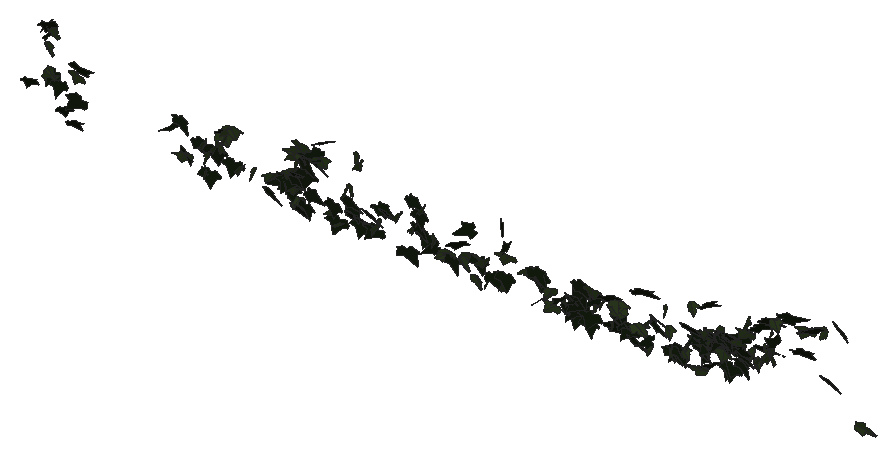
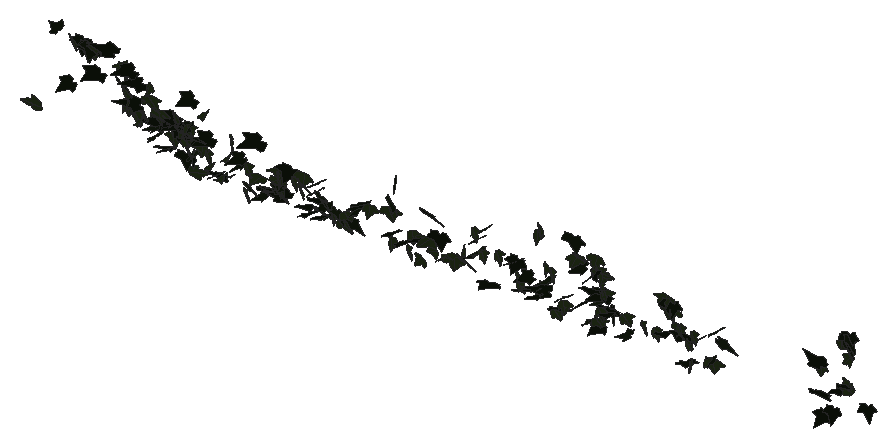
# SketchUp Ruby script. Lengths in millimetres.
U = 1.mm
M = Sketchup.active_model
def pt(a) = Geom::Point3d.new(a.map { |v| v * U })
def face(e, loops, mat)
  f = e.add_face(loops[0].map { |a| pt(a) })
  loops[1..].each { |l| e.add_face(l.map { |a| pt(a) }).erase! }
  f.material = f.back_material = mat if mat
  f
end
# faces: each face lists its corners as indices into pts; further lists are holes
def faces(e, pts, list, mat = nil) = list.each { |f| face(e, (f[0].is_a?(Array) ? f : [f]).map { |l| l.map { |i| pts[i] } }, mat) }
# xy, xz, yz: faces in a plane at the given z, y or x. An outline is a flat list of corners, or four numbers for a rectangle; further outlines are holes
def ring(l) = l.size == 4 ? [[l[0], l[1]], [l[2], l[1]], [l[2], l[3]], [l[0], l[3]]] : l.each_slice(2).to_a
def flat(e, list, mat, &to3) = list.each { |f| face(e, (f[0].is_a?(Array) ? f : [f]).map { |l| ring(l).map { |u, v| to3.(u, v) } }, mat) }
def xy(e, z, list, mat = nil) = flat(e, list, mat) { |x, y| [x, y, z] }
def xz(e, y, list, mat = nil) = flat(e, list, mat) { |x, z| [x, y, z] }
def yz(e, x, list, mat = nil) = flat(e, list, mat) { |y, z| [x, y, z] }
def lines(e, pts, list) = list.each { |a, b| e.add_line(pt(pts[a]), pt(pts[b])) }
# prism: a flat outline (further loops are holes) pulled along v
def prism(e, loops, v, mat = nil)
  f = face(e, loops, mat); d = Geom::Vector3d.new(v.map { |x| x * U })
  f.pushpull(f.normal.samedirection?(d) ? d.length : -d.length)
end
def box(e, o, s, mat = nil) = prism(e, [[o, [o[0] + s[0], o[1], o[2]], [o[0] + s[0], o[1] + s[1], o[2]], [o[0], o[1] + s[1], o[2]]]], [0, 0, s[2]], mat)
def at(x, y, z, deg = 0) = Geom::Transformation.translation(pt([x, y, z])) * Geom::Transformation.rotation(ORIGIN, Z_AXIS, deg.degrees)
def axes(o, x, y, z) = Geom::Transformation.new([*x, 0, *y, 0, *z, 0, *pt(o).to_a, 1])
def part(name) = M.definitions.add(name)
# library, detail: a bought-in or finely detailed component or shape, given as its bounding box
def library(name, o, s) = part(name).tap { |d| box(d.entities, o, s) }
def detail(e, o, s) = box(e.add_group.entities, o, s)
def put(e, d, t, mat = nil) = e.add_instance(d, t).tap { |i| i.material = mat if mat }
def group(e, t, mat = nil) = e.add_group.tap { |g| g.transformation = t; g.material = mat if mat }.entities
root = M.entities
M.materials.add("efeu1").color = [18, 25, 13]
M.materials.add("efeu2").color = [43, 57, 29]
c1 = part("ivyleaf_9")
p = [[39.1,54.8,31.7],[34.5,51.8,30.2],[-5.3,25.2,17.3],[-17.9,28.3,20.9],[-21.6,21.7,17],[-20.2,4.3,5.3],
  [-22.9,-0.3,2.5],[-17.1,-4,-0.6],[-2,-2.1,-1.2],[-0.7,-15.4,-10.1],[16.6,-22.3,-16.7],[21.1,-15.1,-12.5],
  [32.7,-10.7,-11],[46.1,-1.8,-6.6],[30.8,11.2,3.8]]
faces(c1.entities,p,[[0,1,2,3,4,5,6,7,8,9,10,11,12,13,14]],"efeu1")
c2 = part("ivyleaf_10")
p = [[0,12.8,-0.8],[-1.5,51.3,-10.9],[-4.9,51,-11.6],[-13.6,26.5,-7.3],[-13.2,15.9,-4.6],[-21.1,19.3,-7.2],
  [-29.5,16.3,-8.3],[-29.2,8.3,-6.2],[-19.7,-9.8,0.5],[-7.6,-13,4],[1,-12.2,5.8],[-0.4,51.1,-11.1],
  [-1.5,51.1,-10.9],[1,-12.4,5.9],[16.9,-12.4,3.5],[35.1,9.1,-5.1],[35,12.9,-6.1],[20.5,16.4,-4.9],
  [15.8,15,-3.8],[15.3,27.6,-7.1],[12.8,31.3,-7.8]]
faces(c2.entities,p,[[0,1,2,3,4,5,6,7,8,9,10],[11,12,0,13,14,15,16,17,18,19,20]],"efeu2")
put(root,c1,axes([3524.8,853.8,2688.6],[-0.38243,-1.02571,-0.0328],[-0.02604,0.0361,-1.04501],[1.95296,-0.20038,-0.02036]))
put(root,c2,axes([2249.2,836.8,2987.3],[-1.94583,0.29815,0.06081],[-0.10761,0.02331,-1.06497],[-0.56904,-1.02394,-0.00654]))
put(root,c2,axes([2960.6,842.6,2771.6],[-0.10375,-1.04241,-0.06639],[0.01698,0.06602,-1.04382],[1.98787,-0.05497,0.00545]))
put(root,c2,axes([5163.4,847,2805.5],[0.54884,-1.01393,0.11412],[0.04034,-0.11261,-1.05409],[1.94147,0.28897,-0.01036]))
put(root,c2,axes([3837.8,845,2630.1],[-1.522,0.00914,0.62017],[-1.11726,-0.33774,-0.75202],[0.38097,-0.95398,0.27218]))
put(root,c1,axes([3781,843.8,2662.2],[-0.77409,0.78081,-0.50896],[0.22007,-0.50875,-0.87289],[-1.76015,-0.40699,0.1147]))
put(root,c2,axes([2371.2,839.1,2946.3],[-1.56462,-0.61552,-0.30437],[0.59717,0.08559,-1.02058],[1.16244,-0.87245,0.11462]))
put(root,c1,axes([1819.8,855.8,2726.1],[-1.01559,-0.89248,-0.01376],[0.03018,0.00655,-1.03979],[1.69851,-0.53376,0.01024]))
put(root,c2,axes([5434.7,847.5,3054.3],[-1.65245,-0.47011,0.42813],[-0.52953,-0.37065,-0.97126],[1.08812,-0.8943,0.1775]))
put(root,c2,axes([2181.7,847.8,2815.4],[-0.62496,-0.9717,0.2211],[-0.05333,-0.22369,-1.02474],[1.89586,-0.32661,0.04406]))
put(root,c2,axes([840.3,839.1,2880.5],[-1.78166,0.36905,0.24353],[-0.53454,-0.05592,-0.99491],[-0.64994,-0.96568,0.15068]))
put(root,c2,axes([4806.6,848.5,2828],[-0.5462,-0.98923,0.23334],[-0.03803,-0.23693,-1.02901],[1.934,-0.28404,0.04567]))
put(root,c1,axes([5480,827.7,3079.3],[0.8704,0.9826,-0.02659],[-0.005,-0.02811,-1.08378],[-1.87077,0.45725,-0.00947]))
put(root,c2,axes([2720.9,851.5,2683.4],[0.06731,-0.98215,0.34089],[-0.00137,-0.34111,-0.98271],[1.97861,0.03318,-0.01228]))
put(root,c1,axes([4776.2,863.7,2677.8],[-0.34733,-0.64065,0.78184],[-0.14186,-0.78379,-0.65964],[1.91851,-0.17394,0.09277]))
put(root,c1,axes([3188,853.2,2671.4],[0.18907,-1.04431,-0.03336],[-0.04427,0.03129,-1.04883],[1.98806,0.10002,-0.02018]))
put(root,c1,axes([3320.6,844.8,2878.5],[-1.86535,0.38799,0.10195],[-0.1859,0.03022,-1.05409],[-0.74052,-0.98494,0.00782]))
put(root,c2,axes([1658.5,854.2,2723.5],[0.29167,-0.92037,0.46601],[0.22757,-0.45211,-0.93222],[1.95015,0.19041,0.03908]))
put(root,c2,axes([2741.6,841.1,2718.1],[0.53876,-0.97275,-0.25324],[-0.0295,0.25883,-1.01157],[1.91281,0.27797,0.05573]))
put(root,c2,axes([4220.5,854.1,2678.7],[0.20291,-0.93081,0.4596],[0.20811,-0.44938,-0.93547],[1.96471,0.14373,0.05162]))
put(root,c2,axes([4092.2,838.4,2805.9],[-1.96075,0.12903,0.14532],[-0.26905,0.04033,-1.03805],[-0.25379,-1.03965,-0.02224]))
put(root,c2,axes([5231.5,838.5,3036.9],[0.50163,1.03539,0.09613],[0.01258,0.0975,-1.06827],[-1.97899,0.26307,0.01758]))
put(root,c2,axes([5130.2,848.4,2783.3],[0.12425,-1.04507,0.14266],[0.00203,-0.14286,-1.04708],[2.00742,0.06483,-0.00777]))
put(root,c1,axes([721.9,857.1,2788],[-0.70151,-0.91712,-0.02718],[0.01443,0.02467,-1.08247],[1.11929,-0.57512,-0.00308]))
put(root,c1,axes([4004.6,854,2708.3],[-1.90405,-0.31834,0.02077],[-0.03708,-0.00727,-1.04987],[0.60602,-1.00064,0.00102]))
put(root,c2,axes([2524.7,841.7,2817.8],[0.33537,-1.02725,-0.2257],[0.01394,0.23004,-1.04128],[2.00165,0.17051,0.04506]))
put(root,c1,axes([5297.4,834.8,3075.8],[0.5679,-0.01909,1.03753],[1.97495,0.00564,-0.29834],[-0.00027,1.07957,0.0199]))
put(root,c1,axes([3964,856.5,2655.2],[-1.79592,-0.22886,-0.35753],[0.77032,-0.22235,-0.92594],[0.24355,-0.98429,0.2923]))
put(root,c2,axes([1769.1,844.1,2856.5],[0.40161,-1.0348,-0.11686],[0.03197,0.12261,-1.05532],[1.9817,0.20773,0.04071]))
put(root,c1,axes([2359.5,840.3,2956],[-1.405,0.61644,0.46097],[-0.92564,0.12149,-0.94136],[-1.13547,-0.86181,0.19702]))
put(root,c2,axes([5084.8,850.5,2813.4],[1.0935,-0.85291,0.23371],[0.30636,-0.17319,-1.02776],[1.65499,0.59561,0.03583]))
put(root,c1,axes([4909,855.7,2835.7],[0.28184,-1.02702,0.11184],[0.02485,-0.11111,-1.03764],[1.96603,0.14864,-0.00292]))
put(root,c1,axes([4766.3,858.5,2671.6],[-0.31118,0.09515,-1.0236],[1.52436,-0.63795,-0.18724],[-1.2265,-0.81702,0.02699]))
put(root,c2,axes([4706.2,841.7,2943.8],[0.18012,1.06557,-0.0634],[-0.03404,-0.06206,-1.06969],[-2.03129,0.09553,0.0123]))
put(root,c2,axes([3546,844.5,2807.2],[-1.80956,-0.35541,0.30029],[-0.49786,-0.15666,-1.01368],[0.73233,-0.98471,0.05289]))
put(root,c2,axes([3423.7,846,2629.2],[0.49046,-1.02396,-0.05486],[-0.00527,0.05587,-1.05584],[1.95159,0.25749,0.01093]))
put(root,c2,axes([4147.6,844.8,2765.4],[0.29206,-1.03516,-0.1201],[-0.05918,0.11679,-1.04638],[1.98245,0.15599,-0.01354]))
put(root,c1,axes([4835.8,831.1,2659.2],[0.53256,0.98286,-0.06512],[-0.06187,-0.05844,-1.02181],[-1.87366,0.28129,0.01523]))
put(root,c1,axes([2742.9,834.6,2799.4],[1.77656,0.12528,-0.48402],[-0.92454,-0.01528,-0.9408],[-0.22513,1.05137,0.04401]))
put(root,c1,axes([4952.1,859.3,2674.2],[-1.41903,-0.72291,-0.02914],[0.26822,-0.10407,-1.02405],[1.35058,-0.73888,0.17275]))
put(root,c1,axes([2478,857,2633.5],[-1.34236,-0.72939,-0.04705],[0.06489,0.03248,-1.01463],[1.38954,-0.70614,0.00193]))
put(root,c2,axes([4772.1,849.8,2593],[-0.5713,0.16608,-0.97809],[-1.87241,-0.18152,0.27112],[-0.24333,1.00689,0.21021]))
put(root,c2,axes([649.1,847.9,2983.9],[-0.91633,0.44988,-0.67449],[0.65762,-0.40971,-0.87353],[-0.73885,-0.92261,0.05902]))
put(root,c1,axes([4826.2,858.9,2792.3],[-0.76048,0.05698,-0.9592],[1.5315,-0.54789,-0.36777],[-0.99945,-0.88292,0.16631]))
put(root,c2,axes([4900.9,844,2746.7],[1.93704,-0.15175,-0.03007],[-0.00635,0.17855,-1.01386],[0.29435,1.00245,0.17603]))
put(root,c1,axes([4827,856.9,2759.9],[-1.70999,-0.50276,0.04313],[-0.08161,-0.0117,-1.02953],[0.95689,-0.89944,-0.01072]))
put(root,c1,axes([4770.9,852.1,2779.7],[-1.97824,-0.02307,0.01489],[-0.02887,0.01257,-1.03961],[0.04356,-1.03946,-0.01291]))
put(root,c1,axes([5242.8,828.7,2918],[-0.55871,0.81079,0.61449],[-0.48403,0.56077,-0.86141],[-1.87473,-0.38642,0.03927]))
put(root,c1,axes([4938.1,860.7,2666.4],[-0.47857,-0.98898,0.18704],[-0.00593,-0.19202,-1.01951],[1.91558,-0.24767,0.04357]))
put(root,c1,axes([3713.3,848.5,2787.9],[0.13317,-0.99633,-0.43816],[0.23105,0.44347,-0.98902],[2.05856,0.01468,0.13935]))
put(root,c1,axes([3991.1,855.7,2759],[0.10791,-1.02927,-0.01108],[0.05026,0.01255,-1.03047],[1.95837,0.05639,0.02705]))
put(root,c1,axes([4107.5,850.2,2772.3],[-1.68755,0.40318,-0.38442],[0.62497,-0.20543,-0.97289],[-0.85644,-0.94435,0.04751]))
put(root,c2,axes([4101,847.7,2732.1],[0.95268,-0.93252,-0.02492],[0.06155,0.04561,-1.05719],[1.77434,0.49911,0.05005]))
put(root,c1,axes([2982.2,860,2843.2],[-0.18743,-1.02006,0.18085],[-0.04885,-0.17921,-1.02477],[1.97105,-0.10144,-0.0082]))
put(root,c2,axes([5195.3,843.9,2825.3],[-0.33655,-1.03716,-0.15633],[-0.0239,0.16062,-1.0514],[1.99607,-0.17295,-0.03895]))
put(root,c2,axes([2600.2,841.7,3040.9],[0.94944,-0.8955,-0.3093],[-0.00123,0.34923,-1.01217],[1.80311,0.47177,0.16217]))
put(root,c1,axes([4051.6,857.4,2615],[-0.36566,-1.02505,-0.02846],[-0.01091,0.03003,-1.04284],[1.9516,-0.19189,-0.01117]))
put(root,c1,axes([4801.8,823.6,2981.8],[1.0595,0.6289,0.69898],[0.9003,0.51468,-0.83983],[-1.54653,0.73046,-0.01005]))
put(root,c1,axes([652.9,837.1,3113],[0.67461,0.83088,-0.50179],[-0.36156,-0.4054,-0.99787],[-1.12764,0.62706,0.01976]))
put(root,c2,axes([1866.2,849,2717],[-0.03693,-1.03805,0.06821],[-0.02331,-0.06799,-1.03817],[1.97974,-0.02017,-0.01095]))
put(root,c2,axes([4892.9,847.5,2866],[1.19897,-0.85151,-0.01828],[0.14211,0.07787,-1.05387],[1.61473,0.62541,0.10632]))
put(root,c2,axes([1631.8,847.4,2777.5],[0.15517,-1.04614,-0.0366],[0.00203,0.0368,-1.0493],[1.99223,0.08144,0.00392]))
put(root,c2,axes([1756.2,841.6,2862.7],[1.74782,0.41459,0.34556],[0.49005,0.26283,-0.99965],[-0.90276,0.94536,0.12638]))
put(root,c1,axes([847.3,856.1,2736.8],[-1.85697,-0.29641,0.05056],[-0.09128,-0.01608,-1.01974],[0.56495,-0.97689,0.00144]))
put(root,c1,axes([3521.7,825,2971],[0.1987,0.34296,-1.03239],[-1.72012,0.60458,0.10944],[1.15234,0.84333,0.34139]))
put(root,c2,axes([1803.7,839.9,2920.1],[1.88423,0.20389,0.3712],[0.53319,0.3925,-0.9628],[-0.60447,0.98179,0.30782]))
put(root,c1,axes([4205.4,837.6,2644.7],[0.56789,-0.08644,1.07907],[2.06015,0.01167,-0.29839],[0.02237,1.11951,0.08643]))
put(root,c2,axes([4996.3,843.5,2842.1],[-1.85555,0.00075,0.3707],[-0.70424,-0.06486,-0.97306],[0.04254,-1.04104,0.0609]))
put(root,c1,axes([4804.2,848.2,2828.9],[1.39993,-0.75627,0.08125],[0.24801,0.01394,-1.04997],[1.42622,0.73991,0.10283]))
put(root,c1,axes([5385.1,832,2928.8],[1.87767,0.38759,0.22071],[0.39423,0.07633,-1.05998],[-0.75178,1.00809,-0.0046]))
put(root,c2,axes([4556.7,848.4,2753.1],[0.18081,1.01006,-0.29537],[0.01311,-0.29716,-1.01397],[-2.00281,0.08924,-0.0333]))
put(root,c1,axes([4173.6,832.4,2808.1],[1.51407,0.6998,-0.06753],[-0.0701,-0.06035,-1.05932],[-1.33621,0.79612,-0.02094]))
put(root,c1,axes([2551.6,844.9,2695.3],[1.4633,-0.37434,0.60056],[1.13248,-0.13804,-0.84783],[0.72903,0.9658,0.11159]))
put(root,c2,axes([4237.1,845.3,2787.7],[1.5894,0.66517,-0.01359],[-0.11775,0.05593,-1.06448],[-1.26073,0.83336,0.08228]))
put(root,c1,axes([1470.1,854.8,2854.2],[0.38581,-1.02413,-0.08631],[-0.00857,0.08709,-1.04393],[1.95602,0.20238,0.01245]))
put(root,c1,axes([2710.6,864.3,2657.9],[-1.4816,-0.58663,0.29971],[-0.15276,-0.37605,-0.94453],[1.24441,-0.74461,0.24089]))
put(root,c1,axes([2967.4,852.3,2779.4],[0.72248,-0.97219,-0.12719],[-0.05329,0.12558,-1.04349],[1.86527,0.38015,0.01945]))
put(root,c2,axes([3251.8,854.7,2685.9],[-1.07715,0.43778,-0.75759],[0.86821,-0.62229,-0.7004],[-1.42103,-0.71205,0.14633]))
put(root,c2,axes([1939.7,854.3,2723.3],[0.68737,-1.00756,0.23911],[0.16631,-0.22267,-1.07031],[1.96382,0.37152,0.00695]))
put(root,c2,axes([5757.7,846.8,2623.9],[0.2653,-0.05489,1.12507],[2.12837,0.14239,-0.13161],[-0.25651,1.12469,0.07157]))
put(root,c2,axes([2489.2,855.6,2610.1],[-0.46165,-0.89885,0.38975],[-0.08079,-0.3915,-0.9293],[1.86284,-0.23973,0.05628]))
put(root,c1,axes([5551,840,2820.8],[1.99954,-0.28673,-0.22437],[-0.38922,0.10217,-1.08816],[0.57328,1.06944,0.0438]))
put(root,c2,axes([5054.3,846.8,2903.5],[-1.65578,-0.20003,0.54473],[-1.00179,-0.14123,-0.89254],[0.46493,-1.0167,0.01681]))
put(root,c1,axes([4901.1,837.5,2851.5],[2.00867,0.1427,-0.16912],[-0.31404,-0.0416,-1.06485],[-0.28059,1.06807,-0.01888]))
put(root,c2,axes([2857.7,849.7,2801.7],[-0.09278,-1.04773,0.01676],[0.02837,-0.01747,-1.04875],[1.9941,-0.0485,0.0157]))
put(root,c2,axes([5208.8,846.6,2895.4],[1.27296,-0.79938,-0.1908],[-0.06895,0.21709,-1.03651],[1.56261,0.66079,0.1097]))
put(root,c1,axes([4065.8,862.1,2653.8],[-1.2522,-0.79879,0.01773],[0.12516,-0.07703,-1.03005],[1.51547,-0.65366,0.09972]))
put(root,c1,axes([3091.1,849.7,2701.1],[-1.7001,0.47822,-0.14667],[0.20459,-0.10964,-1.01222],[-0.92975,-0.89858,0.04545]))
put(root,c1,axes([3970.3,862.3,2625.4],[-0.7348,-0.95523,0.09098],[-0.00188,-0.09768,-1.02969],[1.82622,-0.38445,0.03555]))
put(root,c2,axes([2197.9,839.9,2912.1],[-0.67537,-0.86746,-0.47866],[0.40694,0.4294,-0.93671],[1.84118,-0.41311,0.03145]))
put(root,c1,axes([2312.5,848,2918.4],[1.51589,-0.69692,-0.08546],[-0.11258,0.06217,-1.05832],[1.33155,0.79865,0.00781]))
put(root,c1,axes([4977.3,841.4,2793.4],[0.43064,0.09525,-1.03432],[1.52589,0.65699,0.2359],[1.25681,-0.83029,0.068]))
put(root,c2,axes([2212.4,846.9,2856.8],[0.44043,-1.01871,-0.1879],[-0.04046,0.18782,-1.04446],[1.9711,0.23148,0.02055]))
put(root,c1,axes([4848.1,857.2,2798],[-1.67592,-0.12919,-0.52249],[1.01319,-0.0616,-0.88199],[0.15078,-1.02206,0.1192]))
put(root,c1,axes([2390.5,832.5,3050],[0.56887,1.03665,-0.02085],[-0.32189,0.02734,-1.0654],[-1.94692,0.29838,0.17005]))
put(root,c1,axes([5443.3,833.2,3063.6],[0.59201,1.0353,-0.02549],[-0.04944,-0.0188,-1.08084],[-1.97035,0.31154,0.01946]))
put(root,c1,axes([4883.3,851.7,2828.8],[0.66188,-0.96398,-0.24228],[-0.00401,0.25597,-1.02145],[1.89169,0.33783,0.08261]))
put(root,c2,axes([1709.6,850.8,2786.3],[0.07885,-1.05163,0.02218],[-0.06371,-0.0235,-1.05188],[2.00089,0.04069,-0.03437]))
put(root,c2,axes([4683.4,848.8,2723.5],[0.26435,-1.04108,-0.08736],[0.04998,0.09158,-1.04962],[1.98773,0.13615,0.03801]))
put(root,c1,axes([2144.5,835.2,2738.1],[0.62374,-0.16783,-0.99526],[-1.7124,0.42556,-0.36805],[0.87039,0.95752,-0.01087]))
put(root,c1,axes([3982,830.4,2719.8],[-0.28066,0.85178,0.56979],[-0.37015,0.54193,-0.86048],[-1.91493,-0.2296,0.08282]))
put(root,c2,axes([4542.2,843.7,2859.6],[0.70772,-0.92594,-0.35762],[-0.01438,0.37924,-0.98978],[1.88907,0.34978,0.12645]))
put(root,c1,axes([4673.7,841.3,2812.7],[2.10002,-0.18849,-0.00836],[-0.01636,-0.00064,-1.1194],[0.35872,1.10345,-0.00208]))
put(root,c1,axes([2256.4,848.3,2894.6],[0.78631,-0.87903,-0.41991],[-0.39191,0.367,-0.97089],[1.81216,0.46079,-0.02777]))
put(root,c1,axes([671.4,841.4,3062],[-0.7447,0.92163,0.02249],[-0.01308,0.01987,-1.10544],[-1.12465,-0.6105,-0.00204]))
put(root,c1,axes([2652.5,846,2745.4],[1.80729,-0.4543,0.00246],[0.00416,-0.00113,-1.05268],[0.86462,0.94961,-0.00007]))
put(root,c1,axes([1664.1,858.4,2617.6],[-0.81289,-0.89986,-0.20001],[0.10682,0.19464,-0.99557],[1.75116,-0.42959,-0.03211]))
put(root,c1,axes([3445.8,851.9,2665.5],[0.09104,-0.93068,-0.40341],[0.04437,0.40476,-0.93103],[1.93,0.0346,0.04044]))
put(root,c1,axes([3738.7,859.5,2761.5],[-0.43238,-1.00478,-0.11456],[0.00128,0.11726,-1.02984],[1.92469,-0.2258,-0.02505]))
put(root,c2,axes([3087.1,830.2,2741],[0.16616,-0.3789,-0.99376],[0.00935,0.99724,-0.37979],[2.02412,0.0265,0.08333]))
put(root,c1,axes([2166.9,860.9,2748],[-1.79715,-0.38036,-0.19061],[0.43437,-0.06128,-1.00838],[0.68335,-0.96137,0.13969]))
put(root,c2,axes([2232.1,847.6,2926.5],[0.48052,-0.01406,-1.02872],[-1.9235,0.19468,-0.25071],[0.36614,1.0412,0.03298]))
put(root,c1,axes([3908.6,851.5,2654.7],[0.8191,-0.89576,-0.24795],[-0.10644,0.24779,-0.99226],[1.76572,0.43047,0.05521]))
put(root,c1,axes([2436.9,866.6,2705.3],[-0.41557,-0.93375,0.34678],[0.05145,-0.36044,-0.95351],[1.89501,-0.19498,0.10193]))
put(root,c1,axes([809.7,834.7,2608.9],[1.17742,0.53396,0.01127],[0.00156,0.02097,-1.10282],[-0.65158,0.96494,0.01773]))
put(root,c2,axes([1507.3,849.2,2666.1],[-1.6402,-0.5295,0.15653],[-0.25516,-0.0808,-1.01148],[1.01941,-0.87218,-0.00132]))
put(root,c2,axes([646.8,842.7,2798.6],[-0.56173,-0.28654,0.95842],[0.99959,0.49729,0.54229],[-0.70017,0.93983,0.00527]))
put(root,c1,axes([4984.6,861.6,2828.7],[-1.81633,-0.18504,-0.36514],[0.75773,-0.20428,-0.93708],[0.18109,-1.00119,0.25868]))
put(root,c2,axes([1779.6,838.6,2902.1],[-0.52914,-0.8168,-0.63572],[0.42555,0.59531,-0.86267],[1.92336,-0.35643,0.01598]))
put(root,c1,axes([4872.7,861.3,2800.9],[0.12611,-0.00026,-1.0344],[1.87427,-0.3171,0.06317],[-0.60229,-0.98682,-0.02002]))
put(root,c1,axes([1505.3,867.7,2667.2],[0.15474,-0.77395,0.66392],[0.14092,-0.65978,-0.7782],[1.93556,0.10991,0.00358]))
put(root,c2,axes([2611.3,844.6,3004.9],[-0.18286,-0.99559,-0.36674],[0.24839,0.35436,-0.99615],[2.00393,-0.13477,0.09001]))
put(root,c1,axes([3983,852.4,2808.2],[0.59922,-0.95105,-0.3112],[0.06258,0.3359,-0.99326],[1.90344,0.28835,0.13063]))
put(root,c2,axes([5204,844.4,2826.5],[-1.13829,0.87599,0.07694],[-0.18955,0.02497,-1.05852],[-1.66284,-0.60251,0.068]))
put(root,c1,axes([3027.9,867.6,2733.8],[-0.80058,-0.86898,0.32729],[-0.14544,-0.32569,-0.96296],[1.76127,-0.42189,0.06925]))
put(root,c2,axes([3527.3,844.6,2641.8],[-0.1877,-0.99063,-0.37102],[0.24309,0.35875,-0.99183],[1.99854,-0.13668,0.08579]))
put(root,c2,axes([4249,855.6,2727.9],[0.96642,0.551,0.72978],[-0.95919,-0.52789,0.74925],[1.45216,-0.71538,0.00922]))
put(root,c2,axes([4728,844.4,2752.3],[-1.72191,0.44109,0.26771],[-0.5256,0.0425,-1.00335],[-0.82949,-0.94256,0.08004]))
put(root,c2,axes([5210,838.6,2977.8],[0.49631,-0.79806,-0.66927],[0.09269,0.69852,-0.81396],[1.98011,0.16733,0.20586]))
put(root,c1,axes([4871.9,841.4,2827.5],[1.99021,-0.05683,0.01946],[0.04192,0.04717,-1.04615],[0.10636,1.04484,0.04829]))
put(root,c1,axes([5000.8,860.7,2713.5],[0.4484,-1.00803,0.0812],[0.04097,-0.07835,-1.03519],[1.92425,0.23656,0.00312]))
put(root,c2,axes([3668.5,844.9,2777.2],[-0.92039,-0.88252,-0.33517],[0.25851,0.30762,-1.00597],[1.77797,-0.50157,-0.02724]))
put(root,c2,axes([646.6,852.7,2839.1],[0.71855,0.00063,0.92492],[1.12834,0.01136,-0.58895],[-0.0121,1.09647,0.00557]))
put(root,c1,axes([533.7,843.3,2750.5],[0.69157,0.68354,-0.59156],[-0.52765,-0.40807,-0.88596],[-0.96843,0.71046,0.06028]))
put(root,c2,axes([3394,850,2729],[-0.57532,-1.00367,-0.10117],[0.05423,0.09708,-1.04821],[1.9191,-0.30363,-0.00071]))
put(root,c1,axes([651.9,840,3098.9],[-0.44414,1.05527,0.03181],[-0.01002,0.03081,-1.1163],[-1.28798,-0.36413,-0.00228]))
put(root,c2,axes([686.3,853.4,3050.2],[-1.26648,0.08365,0.31829],[0.38712,-0.02495,1.04146],[0.10649,1.08551,-0.00059]))
put(root,c1,axes([4560.5,856.2,2639],[0.32551,-0.97793,-0.23774],[0.35831,0.26798,-0.96689],[1.8816,0.11815,0.22525]))
put(root,c1,axes([2908.4,851.1,2621.6],[-0.5751,-0.67484,-0.7262],[0.67153,0.63626,-0.73808],[1.76319,-0.46244,0.04424]))
put(root,c1,axes([2931.5,848.5,2918.2],[0.9003,-0.82541,-0.45997],[-0.10371,0.4897,-0.93481],[1.79538,0.44219,0.17665]))
put(root,c1,axes([2261.2,866.6,2637.8],[-0.01569,-0.96592,0.32251],[0.0971,-0.32251,-0.96461],[1.93567,0.00835,0.051]))
put(root,c2,axes([5108.9,849.9,2768.9],[-0.09214,1.04429,-0.13892],[0.00272,-0.13901,-1.0454],[-2.005,-0.04818,0.00497]))
put(root,c1,axes([4266.2,847.2,2685.4],[-1.37498,0.73124,0.0075],[-0.01153,0.00456,-1.02794],[-1.39172,-0.72248,0.0011]))
put(root,c2,axes([4583.5,850.4,2634.2],[0.16462,1.01039,-0.14055],[-0.05648,-0.13851,-1.01393],[-1.94066,0.08974,0.01759]))
put(root,c2,axes([4360.7,842.8,2700.7],[1.28384,0.59612,0.56255],[0.68868,0.43713,-0.89713],[-1.3997,0.76185,0.07457]))
put(root,c2,axes([4662.1,844.2,2666.3],[0.03239,1.01449,0.18738],[-0.09641,0.188,-1.01325],[-1.96106,0.00751,0.05291]))
put(root,c1,axes([2180.9,840,2802.4],[1.93757,0.04602,0.24134],[0.44159,0.15818,-1.00893],[-0.15376,1.03425,0.14357]))
put(root,c1,axes([2155.1,856.5,2739],[-1.84482,0.1802,0.34614],[-0.6695,-0.0023,-0.98393],[-0.32149,-1.02927,0.06279]))
put(root,c1,axes([2523.4,847.7,2774.4],[1.21626,-0.7473,-0.39486],[-0.07954,0.46648,-0.95048],[1.60663,0.58882,0.25186]))
put(root,c1,axes([3229.8,841.1,2773.8],[0.73445,0.93418,-0.24925],[-0.19586,-0.22716,-1.01071],[-1.82967,0.3993,0.00814]))
put(root,c1,axes([2736.6,848.4,2805.2],[0.87663,-0.80089,-0.4997],[0.13008,0.58285,-0.87115],[1.79189,0.3495,0.30771]))
put(root,c1,axes([2211,844.8,2622.9],[1.89422,-0.08963,-0.19402],[-0.37175,-0.00644,-0.99903],[0.16506,1.014,-0.0235]))
put(root,c2,axes([4819.5,864.2,2765.5],[-0.03234,-0.87816,0.53969],[0.12691,-0.53957,-0.87586],[1.95759,0.02047,0.0657]))
put(root,c1,axes([1584.3,853.3,2770],[0.6267,-0.91008,-0.37758],[-0.10759,0.38001,-0.96522],[1.87213,0.32649,0.07093]))
put(root,c1,axes([2615.2,866.7,2655.9],[-0.83885,-0.92166,0.0783],[-0.05103,-0.07397,-1.0216],[1.75968,-0.44151,0.0077]))
put(root,c1,axes([1773.1,839.6,2901.7],[0.72361,0.99082,-0.14473],[-0.07499,-0.13989,-1.06118],[-1.90426,0.38202,-0.01321]))
put(root,c2,axes([5058,836.9,2969.7],[-0.07075,-0.63777,-0.85772],[0.22005,0.8508,-0.63764],[2.02229,-0.11489,0.03937]))
put(root,c1,axes([678.5,864.1,2829.8],[-1.1711,-0.43922,-0.12493],[0.15954,0.01423,-1.05483],[0.53378,-0.96791,0.04118]))
put(root,c1,axes([4314.5,863.9,2661.9],[-1.72971,-0.46811,-0.04788],[0.08652,0.01629,-1.02229],[0.89137,-0.90996,0.00632]))
put(root,c1,axes([4316.1,850.3,2624],[1.40195,-0.69796,-0.23578],[-0.12417,0.27031,-1.00401],[1.3966,0.72467,0.14742]))
put(root,c1,axes([3880.6,836.7,2679.1],[-0.14277,0.97908,0.3179],[-0.28437,0.30501,-0.97464],[-1.93839,-0.11686,0.11957]))
put(root,c1,axes([1451.4,856.1,2807.3],[-1.24304,0.71302,-0.37936],[0.04162,-0.47209,-0.92496],[-1.53658,-0.58959,0.28184]))
put(root,c2,axes([4826.8,850.5,2779],[-1.93049,-0.05409,0.16911],[-0.31621,-0.05661,-1.01469],[0.11913,-1.02678,0.04703]))
put(root,c2,axes([3160.1,856.8,2686],[1.35676,0.31821,-0.67189],[-1.27102,-0.13488,-0.77246],[-0.62165,0.97028,0.11297]))
put(root,c1,axes([2164.5,863.2,2711.2],[-0.69741,-0.93447,-0.21815],[0.22605,0.18755,-1.0029],[1.81225,-0.38301,0.04115]))
put(root,c2,axes([4242.4,844,2761.6],[0.75077,-0.78842,-0.58895],[-0.11044,0.61477,-0.86184],[1.86969,0.3529,0.18558]))
put(root,c1,axes([5612.5,871.1,3112.8],[0.32576,-0.7786,0.7468],[0.43917,-0.71222,-0.79544],[2.00576,0.2824,0.05287]))
put(root,c2,axes([2216.7,863.8,2656.4],[-1.15079,-0.67893,0.45613],[-0.04304,-0.55315,-0.85331],[1.55609,-0.5174,0.31373]))
put(root,c2,axes([2555.3,848.8,2842.2],[1.13997,-0.82304,-0.28597],[0.18756,0.40879,-0.97012],[1.64764,0.52291,0.30829]))
put(root,c1,axes([1695.7,859,2760.8],[-1.26877,-0.45262,-0.66713],[1.08798,0.345,-0.80532],[1.08187,-0.87776,0.02749]))
put(root,c1,axes([3926.4,870.2,2686.2],[-0.23812,-0.40963,0.92801],[0.65513,-0.89671,-0.3494],[1.81604,0.26977,0.24773]))
put(root,c1,axes([4458.1,848.8,2753.4],[1.35832,-0.62816,-0.42994],[-0.48636,0.35743,-0.94643],[1.36464,0.75264,0.09063]))
put(root,c1,axes([2295.2,844.8,2731.1],[0.89929,-0.61408,-0.7153],[-0.27872,0.74259,-0.73425],[1.77243,0.42834,0.24746]))
put(root,c1,axes([3350,862.6,2718.8],[-0.32138,-0.98327,-0.21084],[0.11178,0.20378,-0.9974],[1.91063,-0.17732,0.02289]))
put(root,c1,axes([2267.5,863.7,2816.6],[-1.47227,-0.58488,-0.36776],[0.6431,0.16126,-0.96725],[1.14691,-0.84123,0.07027]))
put(root,c1,axes([2553.3,864.3,2733.8],[0.24712,-1.01833,0.01596],[0.00006,-0.01609,-1.02657],[1.93833,0.12983,-0.002]))
put(root,c1,axes([3732.2,850.9,2749.9],[1.34175,-0.71626,-0.42276],[-0.5484,0.30954,-1.00496],[1.4849,0.76153,0.01086]))
put(root,c1,axes([5426.6,833.9,3058.1],[0.76405,0.95016,0.32318],[0.05701,0.33657,-1.02676],[-1.90923,0.39029,0.09867]))
put(root,c1,axes([4725.3,860.9,2727.8],[0.66935,-0.97481,-0.06017],[0.03078,0.06975,-1.03559],[1.85853,0.34992,0.03882]))
put(root,c1,axes([4439.8,850.2,2638.5],[-1.39343,0.73903,0.00971],[-0.0162,0.00523,-1.04029],[-1.40654,-0.7322,0.00237]))
put(root,c1,axes([2182.7,855.7,2779.4],[0.94666,-0.88998,-0.24287],[0.02442,0.28257,-1.00918],[1.75557,0.47597,0.145]))
put(root,c2,axes([2047.4,862,2735.3],[-0.60199,-0.90197,0.36508],[-0.16491,-0.35625,-0.95523],[1.84455,-0.32622,0.03375]))
put(root,c2,axes([3333.2,857.7,2606.6],[1.38136,-0.56514,0.47445],[1.09025,0.01206,-0.86196],[0.8852,0.86704,0.32124]))
put(root,c1,axes([5170.5,838.4,3018.9],[1.52814,0.40631,0.56612],[0.98686,0.22863,-0.89952],[-0.88598,0.95547,-0.02549]))
put(root,c1,axes([748.3,843.9,2662.1],[0.74958,0.79835,-0.297],[-0.20805,-0.2435,-1.00732],[-1.01816,0.63751,-0.01282]))
put(root,c2,axes([3897.6,850.7,2662.2],[0.9042,-0.85711,-0.33513],[-0.00837,0.37503,-0.9654],[1.75149,0.44427,0.16839]))
put(root,c2,axes([5178.8,833.8,2847.9],[0.20734,-0.01752,-1.05804],[0.14746,1.06091,-0.00959],[2.00853,-0.07608,0.10993]))
put(root,c1,axes([4989.9,858.3,2774.5],[1.0608,-0.87545,-0.09952],[0.09119,0.14771,-1.03096],[1.67441,0.54658,0.1192]))
put(root,c2,axes([4812.9,856.3,2724.4],[0.856,-0.9049,-0.16697],[-0.19016,0.13672,-1.01012],[1.74093,0.45987,-0.02824]))
put(root,c1,axes([4993.3,863.2,2779],[0.37638,-1.00869,-0.13422],[-0.08068,0.12845,-1.02775],[1.93497,0.20156,-0.01675]))
put(root,c2,axes([5532.2,858.3,3078.9],[1.21328,-0.86934,-0.08392],[-0.10748,0.06265,-1.078],[1.65874,0.63994,-0.00847]))
put(root,c2,axes([3297.6,852.1,2725.7],[-1.77796,-0.01619,-0.47853],[0.91051,0.01137,-0.93433],[0.03729,-1.04956,-0.00274]))
put(root,c2,axes([3135,853.8,2675.5],[-1.84937,-0.29226,0.14895],[-0.28624,-0.01691,-1.01436],[0.55481,-0.98292,-0.02683]))
put(root,c1,axes([822.1,863.7,2898.5],[-0.03109,-0.24646,1.0091],[1.48456,-0.66939,-0.15086],[1.30556,0.75529,0.19558]))
put(root,c2,axes([4426.5,859.3,2747.4],[-0.00617,-1.03693,0.03783],[-0.02674,-0.03778,-1.03684],[1.97462,-0.00375,-0.01392]))
put(root,c2,axes([1726.1,852.5,2790.8],[-1.47207,0.70826,0.12326],[-0.39915,-0.04913,-1.03377],[-1.3087,-0.78169,0.17665]))
put(root,c1,axes([2254.9,846.7,2894],[0.07179,-0.47428,0.94553],[-0.17332,0.94116,0.47572],[-2.00576,-0.0983,-0.00727]))
put(root,c1,axes([5125.6,849,2848.5],[1.59122,-0.20903,0.61257],[1.21269,0.09002,-0.83896],[0.21641,1.03255,0.19715]))
put(root,c1,axes([2019.9,860.4,2643.1],[1.1434,-0.8126,0.0376],[0.17034,0.01958,-1.00711],[1.53879,0.60163,0.08355]))
put(root,c1,axes([5118.8,835.9,2967.6],[0.18945,0.53535,-0.92841],[0.2543,0.91894,0.54421],[2.02376,-0.16559,0.01853]))
put(root,c1,axes([3538,834.6,2843.8],[-0.02384,0.65977,0.8441],[0.03859,0.84416,-0.65951],[-2.03864,0.00827,-0.02236]))
put(root,c1,axes([4215.1,855.9,2699],[1.38056,-0.74514,-0.11981],[0.17274,0.2511,-1.01217],[1.42593,0.69101,0.23861]))
put(root,c2,axes([3802.3,864.7,2697.6],[-1.02961,-0.81162,0.33309],[-0.01934,-0.38551,-0.95584],[1.66959,-0.50498,0.19434]))
put(root,c1,axes([4367,840.6,2904.7],[1.90165,0.40498,0.44983],[0.77148,0.19702,-1.07777],[-0.85547,1.07792,0.02798]))
put(root,c1,axes([5060.1,850.7,2877.9],[-1.22491,0.73023,0.38332],[-0.6866,0.18796,-0.96381],[-1.41148,-0.72514,0.13619]))
put(root,c2,axes([3002.5,856.6,2885],[0.08449,-1.03146,-0.17572],[-0.06277,0.17441,-1.03211],[1.99036,0.04928,-0.02509]))
put(root,c1,axes([4618.5,868.7,2649.4],[-1.77909,-0.41363,-0.06479],[0.11642,0.02188,-1.0222],[0.78827,-0.93678,0.00474]))
put(root,c2,axes([2204.1,863.1,2715.6],[-0.42883,-0.99096,0.18723],[0.00015,-0.19187,-1.01538],[1.91936,-0.22139,0.04191]))
put(root,c1,axes([4609.5,868.3,2641.9],[0.02599,-1.02388,-0.05878],[0.06125,0.05919,-1.02344],[1.95089,0.01178,0.03292]))
put(root,c2,axes([4435.1,860.6,2601.8],[0.88582,-0.92877,-0.04513],[-0.00768,0.04845,-1.03871],[1.7697,0.4651,0.01808]))
put(root,c2,axes([1640.1,850.4,2622.7],[0.53828,-0.85179,-0.48721],[0.20457,0.53088,-0.86575],[1.85634,0.18849,0.23668]))
put(root,c2,axes([2437.5,857.5,2671.7],[-0.63264,-0.96187,-0.10175],[0.04498,0.09949,-1.01764],[1.8403,-0.33309,-0.01011]))
put(root,c1,axes([4466.3,851.9,2779.3],[1.8388,-0.36901,-0.14248],[-0.15681,0.18005,-1.02505],[0.73632,0.95987,0.1375]))
